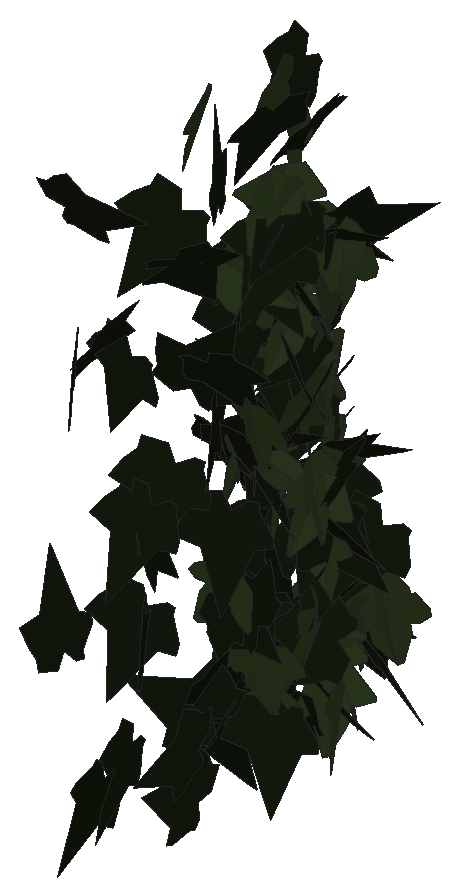
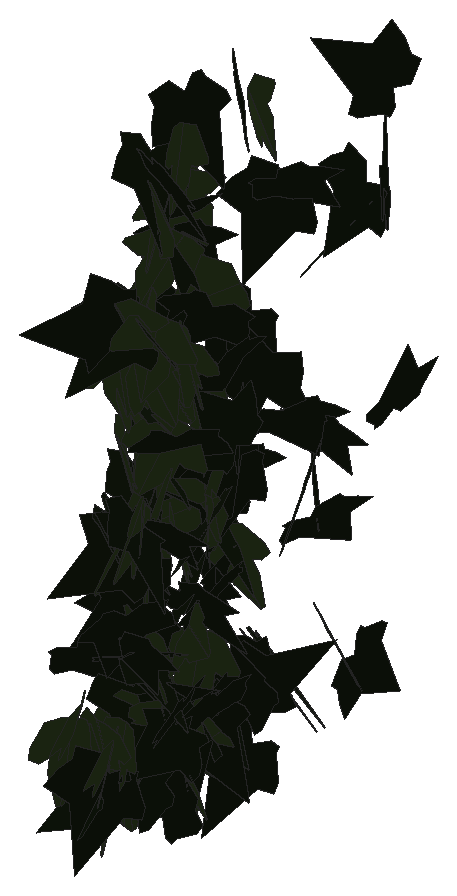
# SketchUp Ruby script. Lengths in inches.
U = 1.inch
M = Sketchup.active_model
def pt(a) = Geom::Point3d.new(a.map { |v| v * U })
def face(e, loops, mat)
  f = e.add_face(loops[0].map { |a| pt(a) })
  loops[1..].each { |l| e.add_face(l.map { |a| pt(a) }).erase! }
  f.material = f.back_material = mat if mat
  f
end
# faces: each face lists its corners as indices into pts; further lists are holes
def faces(e, pts, list, mat = nil) = list.each { |f| face(e, (f[0].is_a?(Array) ? f : [f]).map { |l| l.map { |i| pts[i] } }, mat) }
# xy, xz, yz: faces in a plane at the given z, y or x. An outline is a flat list of corners, or four numbers for a rectangle; further outlines are holes
def ring(l) = l.size == 4 ? [[l[0], l[1]], [l[2], l[1]], [l[2], l[3]], [l[0], l[3]]] : l.each_slice(2).to_a
def flat(e, list, mat, &to3) = list.each { |f| face(e, (f[0].is_a?(Array) ? f : [f]).map { |l| ring(l).map { |u, v| to3.(u, v) } }, mat) }
def xy(e, z, list, mat = nil) = flat(e, list, mat) { |x, y| [x, y, z] }
def xz(e, y, list, mat = nil) = flat(e, list, mat) { |x, z| [x, y, z] }
def yz(e, x, list, mat = nil) = flat(e, list, mat) { |y, z| [x, y, z] }
def lines(e, pts, list) = list.each { |a, b| e.add_line(pt(pts[a]), pt(pts[b])) }
# prism: a flat outline (further loops are holes) pulled along v
def prism(e, loops, v, mat = nil)
  f = face(e, loops, mat); d = Geom::Vector3d.new(v.map { |x| x * U })
  f.pushpull(f.normal.samedirection?(d) ? d.length : -d.length)
end
def box(e, o, s, mat = nil) = prism(e, [[o, [o[0] + s[0], o[1], o[2]], [o[0] + s[0], o[1] + s[1], o[2]], [o[0], o[1] + s[1], o[2]]]], [0, 0, s[2]], mat)
def at(x, y, z, deg = 0) = Geom::Transformation.translation(pt([x, y, z])) * Geom::Transformation.rotation(ORIGIN, Z_AXIS, deg.degrees)
def axes(o, x, y, z) = Geom::Transformation.new([*x, 0, *y, 0, *z, 0, *pt(o).to_a, 1])
def part(name) = M.definitions.add(name)
# library, detail: a bought-in or finely detailed component or shape, given as its bounding box
def library(name, o, s) = part(name).tap { |d| box(d.entities, o, s) }
def detail(e, o, s) = box(e.add_group.entities, o, s)
def put(e, d, t, mat = nil) = e.add_instance(d, t).tap { |i| i.material = mat if mat }
def group(e, t, mat = nil) = e.add_group.tap { |g| g.transformation = t; g.material = mat if mat }.entities
root = M.entities
M.materials.add("efeu1").color = [18, 25, 13]
M.materials.add("efeu2").color = [43, 57, 29]
c1 = part("ivyleaf_9")
p = [[1.54,2.16,1.25],[1.36,2.04,1.19],[-0.21,0.99,0.68],[-0.71,1.11,0.82],[-0.85,0.86,0.67],[-0.8,0.17,0.21],
  [-0.9,-0.01,0.1],[-0.67,-0.16,-0.02],[-0.08,-0.08,-0.05],[-0.03,-0.6,-0.4],[0.65,-0.88,-0.66],[0.83,-0.6,-0.49],
  [1.29,-0.42,-0.43],[1.8125,-0.07,-0.26],[1.21,0.44,0.15]]
faces(c1.entities,p,[[0,1,2,3,4,5,6,7,8,9,10,11,12,13,14]],"efeu1")
c2 = part("ivyleaf_10")
p = [[0,0.5,-0.03],[-0.0625,2.02,-0.43],[-0.19,2.01,-0.46],[-0.54,1.05,-0.29],[-0.52,0.625,-0.18],[-0.83,0.76,-0.28],
  [-1.16,0.64,-0.33],[-1.15,0.33,-0.24],[-0.77,-0.39,0.02],[-0.3,-0.51,0.16],[0.04,-0.48,0.23],[-0.02,2.01,-0.4375],
  [-0.06,2.01,-0.43],[0.04,-0.49,0.23],[0.67,-0.49,0.14],[1.38,0.36,-0.2],[1.375,0.51,-0.24],[0.81,0.65,-0.19],
  [0.62,0.59,-0.15],[0.6,1.09,-0.28],[0.5,1.23,-0.31]]
faces(c2.entities,p,[[0,1,2,3,4,5,6,7,8,9,10],[11,12,0,13,14,15,16,17,18,19,20]],"efeu2")
put(root,c1,axes([53.71,220.875,227.1875],[0.26808,-0.10648,-0.40841],[-0.35175,0.21101,-0.28591],[0.23324,0.44061,0.03823]))
put(root,c1,axes([53.85,223.15,227.02],[0.04386,-0.08728,0.49037],[-0.05575,0.48831,0.0919],[-0.49494,-0.06273,0.03311]))
put(root,c1,axes([53.86,224.08,222.77],[0.25334,-0.21501,0.37362],[-0.28856,0.23736,0.33226],[-0.32024,-0.38397,-0.00383]))
put(root,c1,axes([53.65,223.87,224.12],[0.20708,0.31802,0.32554],[0.13411,0.29914,-0.37753],[-0.43489,0.24368,0.03859]))
put(root,c1,axes([53.69,222.63,227.94],[0.4292,0.14225,-0.21344],[-0.20528,-0.05895,-0.45209],[-0.15378,0.4757,0.0078]))
put(root,c2,axes([53.55,223.93,223.43],[0.36341,-0.25027,0.23515],[0.19509,-0.1313,-0.44125],[0.28261,0.41246,0.00222]))
put(root,c1,axes([53.35,223.14,228.56],[0.12228,-0.24505,0.41833],[0.29297,-0.3064,-0.26512],[0.38629,0.30995,0.06865]))
put(root,c1,axes([53.79,221.55,232],[-0.35244,-0.34591,0.07832],[-0.03217,-0.07879,-0.4927],[0.3532,-0.35234,0.03328]))
put(root,c1,axes([53.85,224.28,233.34],[-0.47178,0.03645,-0.16155],[0.16156,-0.0059,-0.47314],[-0.0364,-0.49863,-0.00621]))
put(root,c2,axes([53.69,223.72,225.65],[-0.03484,0.3885,-0.31282],[-0.02011,-0.31442,-0.38825],[-0.49838,-0.01447,0.03753]))
put(root,c1,axes([53.95,224.66,227.83],[-0.2028,0.45614,-0.0285],[0.00863,-0.02735,-0.49918],[-0.45694,-0.20296,0.00322]))
put(root,c1,axes([53.78,224.55,227.66],[-0.42778,-0.24124,-0.09383],[0.12287,-0.02972,-0.48376],[0.22783,-0.43694,0.08471]))
put(root,c1,axes([53.66,222.41,223.18],[0.44366,0.20798,-0.09955],[-0.09317,-0.03575,-0.48994],[-0.21091,0.45329,0.00704]))
put(root,c1,axes([53.61,223.18,229.74],[-0.00944,-0.49762,0.04776],[-0.00314,-0.04771,-0.49771],[0.4999,-0.0097,-0.00222]))
put(root,c1,axes([53.5625,223.29,224.4],[0.16078,-0.40258,-0.24916],[-0.04154,0.25012,-0.43094],[0.47162,0.15928,0.04699]))
put(root,c2,axes([53.73,223.75,230.24],[0.34952,-0.35611,0.03197],[0.02471,-0.02054,-0.49897],[0.35668,0.35038,0.00324]))
put(root,c2,axes([53.77,224.76,227.9],[0.11792,-0.31917,-0.36636],[0.03356,0.38145,-0.32151],[0.48474,0.05124,0.11138]))
put(root,c1,axes([54.03,221.96,223.76],[-0.01589,0.01203,0.4996],[-0.48102,-0.13592,-0.01203],[0.13552,-0.48102,0.01589]))
put(root,c1,axes([53.92,223.57,226.09],[-0.4826,-0.12619,-0.03426],[0.03245,0.01134,-0.49882],[0.12667,-0.48368,-0.00276]))
put(root,c1,axes([53.55,222.18,228.88],[-0.2227,-0.0518,0.44466],[0.4145,-0.21146,0.18296],[0.1691,0.45011,0.13712]))
put(root,c2,axes([53.76,222.13,233.51],[0.22337,-0.43254,0.11407],[0.04208,-0.10662,-0.48668],[0.44535,0.22702,-0.01123]))
put(root,c1,axes([53.65,223.96,224.54],[0.26329,-0.32578,-0.27303],[-0.17157,0.21239,-0.41887],[0.3889,0.31426,0.00005]))
put(root,c1,axes([53.37,219.6,232.82],[0.18651,-0.14709,0.43998],[0.41146,-0.16658,-0.23011],[0.21427,0.4479,0.0589]))
put(root,c1,axes([53.97,223.17,223.92],[-0.04105,0.36382,-0.34051],[-0.03154,-0.34287,-0.36255],[-0.49731,-0.00829,0.0511]))
put(root,c2,axes([53.83,224.71,227.875],[-0.35992,0.34694,-0.00946],[-0.04489,-0.06005,-0.49435],[-0.34415,-0.355,0.07437]))
put(root,c1,axes([53.75,219.87,223.51],[-0.06608,0.10869,-0.48355],[0.29577,-0.38279,-0.12646],[-0.39769,-0.30275,-0.0137]))
put(root,c2,axes([53.69,223.16,227.54],[0.10129,-0.26683,0.41054],[0.21711,-0.35129,-0.28188],[0.43887,0.23537,0.0447]))
put(root,c1,axes([53.65,223.66,227.04],[0.02814,-0.38757,0.31464],[0.03455,-0.31287,-0.38848],[0.49801,0.04361,0.00917]))
put(root,c1,axes([53.57,223.49,227.31],[0.28699,-0.40531,0.05792],[0.03831,-0.04383,-0.4966],[0.40763,0.28948,0.0059]))
put(root,c2,axes([53.92,225.03,224.375],[-0.45002,0.21117,0.05378],[-0.05796,0.00295,-0.49662],[-0.21006,-0.45321,0.02182]))
put(root,c2,axes([53.9,224.28,230.63],[-0.46484,-0.17847,-0.04554],[0.04139,0.01924,-0.49791],[0.17947,-0.46667,-0.00311]))
put(root,c1,axes([53.93,220.71,227.64],[-0.43137,-0.21602,-0.13138],[0.1321,0.02896,-0.48136],[0.21558,-0.45,0.03209]))
put(root,c2,axes([53.81,223.85,230.2],[0.48677,0.11392,0.00857],[0.00776,0.00447,-0.49992],[-0.11398,0.48683,0.00259]))
put(root,c1,axes([54.03,222.68,223.83],[-0.30815,0.29516,-0.26062],[0.16269,-0.20593,-0.42558],[-0.35857,-0.34709,0.03088]))
put(root,c1,axes([53.75,223.93,228.83],[-0.17134,-0.4148,-0.22042],[0.1383,0.17967,-0.44563],[0.4489,-0.21368,0.05317]))
put(root,c1,axes([53.85,221.9,223.96],[0.11362,0.22955,0.42942],[0.19392,0.38314,-0.25612],[-0.44664,0.22474,-0.00196]))
put(root,c1,axes([53.9,221.29,228.05],[-0.29571,-0.40022,-0.04875],[0.03282,0.03636,-0.49759],[0.40184,-0.29749,0.00476]))
put(root,c2,axes([53.92,224.03,228.08],[-0.27215,0.41692,0.04596],[-0.03353,0.03299,-0.49778],[-0.4181,-0.27403,0.01]))
put(root,c2,axes([54,224.28,230.02],[-0.07086,-0.45609,0.19225],[-0.01322,-0.1924,-0.46131],[0.49478,-0.07046,0.01521]))
put(root,c1,axes([54,219.38,230.88],[0.08406,0.40198,0.28521],[0.06207,0.2784,-0.41066],[-0.48896,0.10444,-0.0031]))
put(root,c1,axes([53.93,220.63,226.05],[-0.20688,-0.4486,0.07719],[-0.02112,-0.07524,-0.49386],[0.4547,-0.20759,0.01218]))
put(root,c1,axes([53.75,222.52,228.49],[-0.0343,-0.04102,-0.49713],[0.44822,-0.22122,-0.01267],[-0.21891,-0.44652,0.05195]))
put(root,c1,axes([53.97,220.23,224.01],[-0.39023,0.04591,-0.30921],[0.30132,-0.0764,-0.39162],[-0.08321,-0.49199,0.03196]))
put(root,c1,axes([53.62,222.81,227.66],[0.27858,0.01576,0.4149],[0.39781,0.13296,-0.27216],[-0.11891,0.48174,0.06154]))
put(root,c1,axes([53.71,223.22,230.65],[-0.04835,-0.28201,-0.41004],[0.23794,0.34873,-0.2679],[0.43709,-0.22104,0.10048]))
put(root,c1,axes([53.78,223.15,225.96],[0.14642,-0.47292,-0.07007],[-0.02182,0.0666,-0.49506],[0.47758,0.14804,-0.00114]))
put(root,c2,axes([53.69,224.28,232.43],[0.02393,-0.08647,-0.49189],[0.32077,-0.37479,0.08149],[-0.3828,-0.31946,0.03753]))
put(root,c1,axes([54.02,224.84,225.83],[-0.43091,-0.18631,-0.17205],[0.15789,0.06837,-0.46947],[0.19846,-0.45893,-0.00009]))
put(root,c1,axes([53.97,225.26,223.82],[0.36581,0.31774,-0.12338],[-0.08312,-0.09237,-0.48431],[-0.33057,0.37484,-0.01476]))
put(root,c2,axes([54.02,223.46,233.36],[0.04597,-0.43989,-0.23319],[0.02176,0.23574,-0.4404],[0.49741,0.03034,0.04082]))
put(root,c1,axes([53.86,224.95,226.32],[-0.06261,-0.44312,-0.22298],[0.03365,0.22044,-0.44752],[0.49492,-0.07104,0.00222]))
put(root,c2,axes([53.99,225.21,224.21],[-0.15075,0.47538,-0.0359],[0.00213,-0.03698,-0.49863],[-0.47673,-0.15049,0.00912]))
put(root,c2,axes([53.96,223.87,228.78],[-0.40715,-0.2187,-0.19079],[0.18887,0.04991,-0.46026],[0.22036,-0.44685,0.04198]))
put(root,c2,axes([53.83,223.15,223.56],[0.22789,0.21854,0.38769],[0.22733,0.31729,-0.31249],[-0.3826,0.3187,0.04525]))
put(root,c1,axes([53.93,220.29,230.27],[-0.03817,-0.41735,0.27269],[0.04227,-0.27522,-0.41529],[0.49675,-0.00865,0.0563]))
put(root,c2,axes([54.14,223.8,229.6],[0.21164,0.38624,-0.2367],[-0.15043,-0.18651,-0.43885],[-0.42729,0.25697,0.03725]))
put(root,c1,axes([54.1,221.14,231.53],[0.28528,0.41054,-0.00842],[-0.00435,-0.00722,-0.49993],[-0.41061,0.28531,-0.00055]))
put(root,c1,axes([53.96,218.95,230.33],[-0.00321,0.14433,0.4787],[0.01035,-0.47859,0.14437],[0.49988,0.01084,0.00008]))
put(root,c1,axes([53.76,224.28,223.39],[0.4266,-0.18664,0.18214],[0.16749,-0.07158,-0.46564],[0.19989,0.4583,0.00145]))
put(root,c2,axes([53.85,223.27,227.45],[-0.26131,-0.10365,-0.41349],[0.42198,0.00588,-0.26814],[0.06045,-0.4891,0.0844]))
put(root,c2,axes([53.93,224.07,224.19],[-0.05801,-0.15622,-0.47141],[0.34012,0.33334,-0.15232],[0.36187,-0.33835,0.06759]))
put(root,c2,axes([54.37,224.41,230.74],[-0.39878,-0.11828,0.27747],[-0.20625,-0.22868,-0.39391],[0.22008,-0.42862,0.13359]))
put(root,c1,axes([54.39,224.04,225.34],[-0.2958,0.38704,-0.11271],[0.02817,-0.11961,-0.48466],[-0.40213,-0.29308,0.04895]))
put(root,c2,axes([54.27,223.89,224.75],[0.32635,-0.3133,-0.21294],[-0.13833,0.16309,-0.45196],[0.35265,0.3539,0.01977]))
put(root,c2,axes([54.09,225.2,224.5],[0.47543,-0.14366,0.05771],[0.054,-0.02078,-0.49664],[0.14509,0.47847,-0.00424]))
put(root,c2,axes([54.125,224.375,223.85],[0.20618,0.45294,-0.04834],[-0.02904,-0.03989,-0.49756],[-0.45459,0.20798,0.00986]))
put(root,c2,axes([54.09,223.53,227.02],[0.34367,-0.3276,0.15675],[0.1224,-0.0987,-0.47463],[0.34192,0.3646,0.01236]))
put(root,c2,axes([54.26,224.68,223.32],[-0.31941,0.35671,0.14398],[-0.09599,0.10732,-0.47882],[-0.37251,-0.33353,-0.00007]))
put(root,c2,axes([53.91,222.65,230.65],[0.20645,0.09588,0.44518],[0.31801,0.31952,-0.21629],[-0.32596,0.37245,0.07095]))
put(root,c2,axes([54.39,221.95,226.04],[0.40731,-0.01228,-0.28974],[-0.2775,0.1286,-0.39555],[0.08423,0.48302,0.09794]))
put(root,c1,axes([54.25,224.15,230.68],[-0.4115,-0.03142,-0.28228],[0.27915,-0.13645,-0.39174],[-0.05242,-0.47999,0.12984]))
put(root,c1,axes([54.4,224.16,224.67],[-0.02187,0.49331,0.07856],[-0.01556,0.07792,-0.49365],[-0.49928,-0.02404,0.01194]))
put(root,c1,axes([54.17,224.61,225.43],[-0.27843,-0.41497,-0.0166],[0.13627,-0.07241,-0.47559],[0.39231,-0.26936,0.15341]))
put(root,c1,axes([54.37,218.22,226.66],[-0.17408,-0.34466,0.31766],[0.14005,0.28513,0.38612],[-0.44731,0.22341,-0.00273]))
put(root,c1,axes([54.05,223.48,225.74],[0.01426,-0.24151,0.43757],[0.07456,-0.43183,-0.24077],[0.4942,0.07211,0.0237]))
put(root,c2,axes([54.375,223.72,226.64],[0.07511,-0.31822,-0.37828],[-0.09047,0.36731,-0.32696],[0.48598,0.11756,-0.0024]))
put(root,c2,axes([54.34,224.67,224.41],[-0.07328,-0.46792,0.16027],[-0.00648,-0.1611,-0.47329],[0.49456,-0.07144,0.01755]))
put(root,c1,axes([54.58,220.94,223.875],[-0.41425,0.27387,0.05827],[-0.04806,0.03296,-0.49659],[-0.27584,-0.41703,-0.00098]))
put(root,c1,axes([54.66,223.98,224.35],[-0.27358,-0.26692,-0.32234],[-0.221,-0.23489,0.38208],[-0.3554,0.35154,0.01054]))
put(root,c1,axes([54.58,222.16,226.71],[-0.31631,0.38631,-0.02672],[0.02041,-0.01781,-0.49927],[-0.38669,-0.31694,-0.0045]))
put(root,c2,axes([54.16,224.25,225.71],[0.46221,-0.02686,0.1888],[0.18925,0.00367,-0.46279],[0.02347,0.49926,0.01356]))
put(root,c2,axes([54.3,224.375,223.3],[0.20049,0.45127,-0.07849],[-0.03494,-0.07036,-0.49379],[-0.45671,0.20349,0.00332]))
put(root,c2,axes([54.42,224.48,230.22],[-0.29207,-0.39745,0.082],[0.01862,-0.11405,-0.48646],[0.4054,-0.28111,0.08142]))
put(root,c1,axes([54.63,223.79,229.28],[-0.42887,0.25207,-0.05031],[-0.00156,-0.10042,-0.48981],[-0.25703,-0.41998,0.08692]))
put(root,c2,axes([54.35,224.24,227.16],[0.06855,-0.26974,-0.41538],[0.08095,0.4198,-0.25925],[0.48862,-0.03171,0.10122]))
put(root,c1,axes([54.21,224.36,227.04],[0.37103,0.22308,0.25015],[0.13548,0.2415,-0.41632],[-0.30657,0.37671,0.11875]))
put(root,c1,axes([54.27,221.67,229.68],[0.44944,0.20915,-0.06531],[-0.05786,-0.03047,-0.49571],[-0.21133,0.45313,-0.00319]))
put(root,c1,axes([54.12,225.33,223.58],[0.41395,-0.27725,0.0422],[0.02799,-0.03403,-0.49806],[0.27905,0.4147,-0.01265]))
put(root,c2,axes([54.46,222.59,224.61],[-0.47228,-0.16099,-0.03211],[0.03321,0.00208,-0.49889],[0.16077,-0.47337,0.00873]))
put(root,c2,axes([54.47,223.36,232.15],[-0.32917,0.35227,0.13249],[-0.0787,0.1077,-0.48188],[-0.36804,-0.33809,-0.01546]))
put(root,c1,axes([54.31,224.22,230.66],[0.4236,0.2603,0.05299],[-0.01614,0.12478,-0.48391],[-0.26515,0.40826,0.11411]))
put(root,c1,axes([54.625,223.43,232.9],[-0.08291,0.49281,0.01613],[0.00282,0.01683,-0.49971],[-0.49307,-0.08278,-0.00557]))
put(root,c1,axes([54.33,221.94,225.82],[0.23042,-0.25345,-0.36424],[-0.17319,0.3265,-0.33675],[0.40855,0.28136,0.06268]))
put(root,c1,axes([54.53,222.89,231.34],[-0.30401,0.24432,-0.31287],[0.2315,-0.21101,-0.38972],[-0.32247,-0.38182,0.01518]))
put(root,c2,axes([54.35,224.4375,228.76],[0.33379,-0.33049,0.17135],[0.13473,-0.1073,-0.4694],[0.34704,0.35953,0.01742]))
put(root,c1,axes([54.07,224.1,226.2],[0.39012,-0.16697,0.26444],[0.23753,-0.11683,-0.42418],[0.20344,0.45659,-0.01183]))
put(root,c1,axes([54.8125,222.04,225.53],[-0.10589,0.18073,0.45401],[-0.27415,0.36258,-0.20827],[-0.40451,-0.29305,0.02231]))
put(root,c1,axes([54.36,223.36,230.38],[0.46002,-0.06479,-0.18489],[-0.18375,0.02106,-0.46454],[0.06798,0.49534,-0.00444]))
put(root,c1,axes([54.19,224.1875,226.05],[-0.03927,-0.10483,-0.48731],[0.31642,0.37245,-0.10562],[0.38514,-0.31669,0.03708]))
put(root,c2,axes([54.56,222.9,232.05],[-0.15974,-0.39753,0.25779],[0.00301,-0.27289,-0.41895],[0.47379,-0.1323,0.08957]))
put(root,c1,axes([54.58,225.1,225.625],[-0.34774,-0.35739,0.03673],[-0.03357,-0.01857,-0.49853],[0.3577,-0.34919,-0.01108]))
put(root,c1,axes([54.47,223.25,229.17],[0.3955,-0.1185,-0.28203],[-0.26872,0.08571,-0.41285],[0.14619,0.47813,0.00411]))
put(root,c1,axes([54.39,219.95,225.71],[-0.0668,0.22708,0.44042],[0.03506,-0.44113,0.23276],[0.49428,0.06198,0.04301]))
put(root,c2,axes([54.48,224.18,229.56],[0.16512,-0.41053,0.23282],[0.10364,-0.20909,-0.4422],[0.46043,0.19429,0.01605]))
put(root,c1,axes([54.72,221.28,232.69],[0.02991,-0.01896,0.49874],[-0.0952,0.49025,0.02435],[-0.48994,-0.09641,0.02572]))
put(root,c1,axes([54.68,222.57,233.49],[-0.08327,0.40836,-0.27623],[0.05551,-0.2706,-0.41677],[-0.48988,-0.10008,-0.00027]))
put(root,c1,axes([54.78,223.35,228.58],[-0.32021,0.38183,-0.04088],[0.03221,-0.02633,-0.49827],[-0.38266,-0.32173,-0.00773]))
put(root,c1,axes([54.77,223.5625,227.74],[-0.14568,0.47342,0.06823],[-0.03293,0.06122,-0.49514],[-0.47717,-0.14876,0.01334]))
put(root,c2,axes([54.43,223.73,224.43],[0.07821,-0.12729,0.47716],[0.24785,-0.40774,-0.14939],[0.42715,0.25989,-0.00068]))
put(root,c1,axes([54.9375,220.51,223.34],[-0.30759,0.30795,0.24609],[-0.17589,0.17212,-0.43524],[-0.35278,-0.35432,0.00244]))
put(root,c1,axes([54.49,221.87,227.24],[-0.14712,-0.47211,-0.07393],[0.02643,0.0692,-0.49448],[0.47713,-0.14941,0.0046]))
put(root,c2,axes([54.6,223.73,226.87],[0.16392,0.38303,-0.27644],[-0.11502,-0.25144,-0.41659],[-0.45815,0.20017,0.00568]))
put(root,c2,axes([54.68,222.1875,228.77],[-0.47955,0.12411,0.06801],[-0.06911,0.00434,-0.49518],[-0.1235,-0.48433,0.01299]))
put(root,c2,axes([54.59,222.95,232.18],[0.15399,0.46934,-0.07749],[-0.09129,-0.05078,-0.48897],[-0.46685,0.16474,0.07006]))
put(root,c2,axes([54.64,225.26,224.26],[-0.33171,-0.36798,-0.06753],[0.05547,0.04088,-0.49523],[0.36999,-0.33604,0.0137]))
put(root,c2,axes([54.49,223.08,231.29],[0.29351,0.29906,0.27279],[0.0688,0.2952,-0.39765],[-0.3989,0.27096,0.13214]))
put(root,c1,axes([54.67,222.875,231.33],[-0.33543,-0.37077,-0.00377],[0.00146,0.00377,-0.49998],[0.37079,-0.33543,-0.00145]))
put(root,c2,axes([54.6,223.62,227.16],[-0.12634,0.48021,-0.05861],[0.00388,-0.05957,-0.49642],[-0.48376,-0.12589,0.01133]))
put(root,c2,axes([54.69,223.3125,228.65],[-0.06144,-0.41607,-0.2704],[0.02261,0.26983,-0.42033],[0.49569,-0.06388,-0.01434]))
put(root,c1,axes([54.51,222.86,223.5],[-0.10363,-0.48841,-0.02669],[0.06334,0.01365,-0.49578],[0.48502,-0.10614,0.05904]))
put(root,c1,axes([54.63,223.16,231.74],[-0.2234,-0.41817,0.15883],[-0.01823,-0.16888,-0.47026],[0.44694,-0.21591,0.06021]))
put(root,c2,axes([54.6,225.2,224.57],[-0.14548,0.47406,-0.06406],[0.03001,-0.05778,-0.49574],[-0.47742,-0.14809,-0.01164]))
put(root,c1,axes([54.42,224.49,230.62],[0.17846,0.12992,0.44863],[0.37492,0.24656,-0.22055],[-0.27854,0.41512,-0.00942]))
put(root,c2,axes([54.71,223.48,230.52],[-0.41197,0.27812,0.05418],[-0.04466,0.03068,-0.49706],[-0.2798,-0.41438,-0.00044]))
put(root,c1,axes([54.875,224.06,227.23],[-0.39392,0.26541,-0.15617],[0.09073,-0.14228,-0.47066],[-0.29427,-0.39914,0.06393]))
put(root,c2,axes([54.52,224.25,223.17],[0.17806,-0.33847,0.32207],[0.24856,-0.22322,-0.37201],[0.39562,0.29259,0.08877]))
